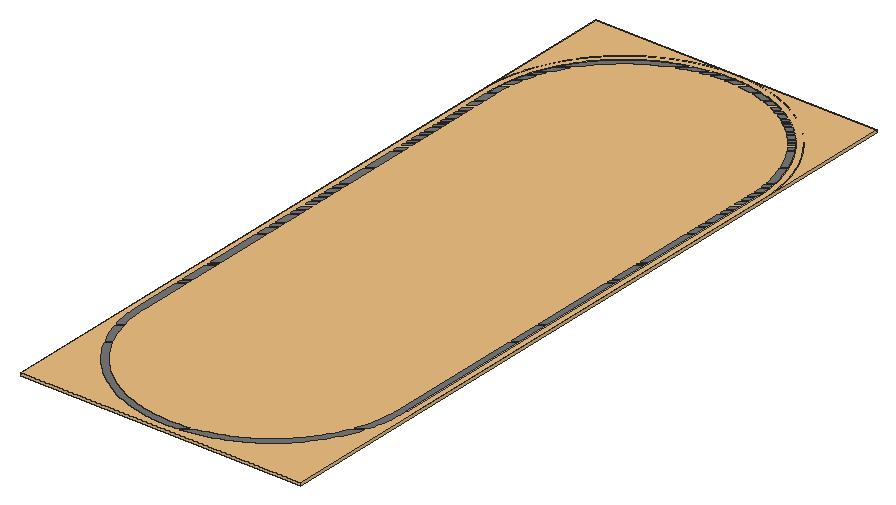
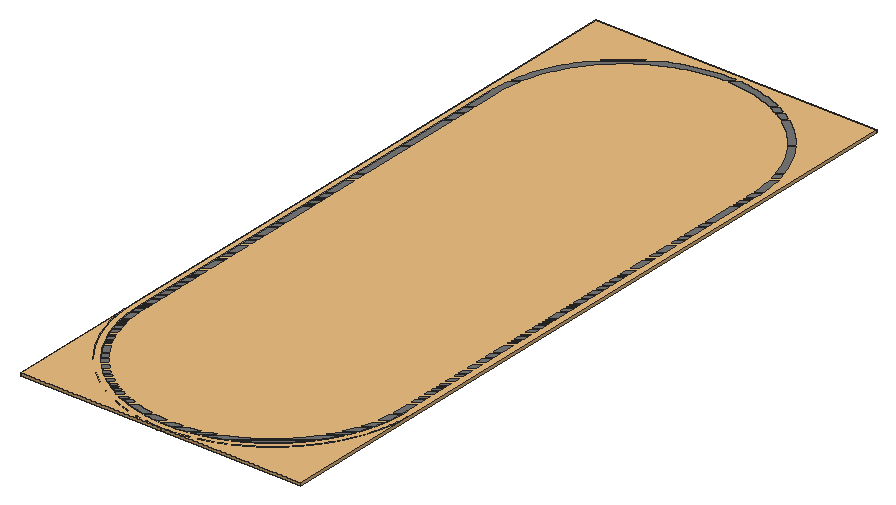
# SketchUp Ruby script. Lengths in inches.
U = 1.inch
M = Sketchup.active_model
def pt(a) = Geom::Point3d.new(a.map { |v| v * U })
def face(e, loops, mat)
  f = e.add_face(loops[0].map { |a| pt(a) })
  loops[1..].each { |l| e.add_face(l.map { |a| pt(a) }).erase! }
  f.material = f.back_material = mat if mat
  f
end
# faces: each face lists its corners as indices into pts; further lists are holes
def faces(e, pts, list, mat = nil) = list.each { |f| face(e, (f[0].is_a?(Array) ? f : [f]).map { |l| l.map { |i| pts[i] } }, mat) }
# xy, xz, yz: faces in a plane at the given z, y or x. An outline is a flat list of corners, or four numbers for a rectangle; further outlines are holes
def ring(l) = l.size == 4 ? [[l[0], l[1]], [l[2], l[1]], [l[2], l[3]], [l[0], l[3]]] : l.each_slice(2).to_a
def flat(e, list, mat, &to3) = list.each { |f| face(e, (f[0].is_a?(Array) ? f : [f]).map { |l| ring(l).map { |u, v| to3.(u, v) } }, mat) }
def xy(e, z, list, mat = nil) = flat(e, list, mat) { |x, y| [x, y, z] }
def xz(e, y, list, mat = nil) = flat(e, list, mat) { |x, z| [x, y, z] }
def yz(e, x, list, mat = nil) = flat(e, list, mat) { |y, z| [x, y, z] }
def lines(e, pts, list) = list.each { |a, b| e.add_line(pt(pts[a]), pt(pts[b])) }
# prism: a flat outline (further loops are holes) pulled along v
def prism(e, loops, v, mat = nil)
  f = face(e, loops, mat); d = Geom::Vector3d.new(v.map { |x| x * U })
  f.pushpull(f.normal.samedirection?(d) ? d.length : -d.length)
end
def box(e, o, s, mat = nil) = prism(e, [[o, [o[0] + s[0], o[1], o[2]], [o[0] + s[0], o[1] + s[1], o[2]], [o[0], o[1] + s[1], o[2]]]], [0, 0, s[2]], mat)
def at(x, y, z, deg = 0) = Geom::Transformation.translation(pt([x, y, z])) * Geom::Transformation.rotation(ORIGIN, Z_AXIS, deg.degrees)
def axes(o, x, y, z) = Geom::Transformation.new([*x, 0, *y, 0, *z, 0, *pt(o).to_a, 1])
def part(name) = M.definitions.add(name)
# library, detail: a bought-in or finely detailed component or shape, given as its bounding box
def library(name, o, s) = part(name).tap { |d| box(d.entities, o, s) }
def detail(e, o, s) = box(e.add_group.entities, o, s)
def put(e, d, t, mat = nil) = e.add_instance(d, t).tap { |i| i.material = mat if mat }
def group(e, t, mat = nil) = e.add_group.tap { |g| g.transformation = t; g.material = mat if mat }.entities
root = M.entities
M.materials.add("False ceiling Light").color = [253, 207, 127]
M.materials.add("[Slate Light Tile]").color = [119, 119, 119]
c1 = library("Group\#44",[0,0,0],[46,118,0.5])
xy(root,3,[[[189,26,189.58,26.01,190.15,26.03,190.73,26.07,191.3,26.12,191.87,26.1875,192.44,26.27,193.01,26.37,193.57,26.48,194.14,26.61,194.69,26.75,195.25,26.91,195.8,27.08,196.34,27.26,196.88,27.46,197.42,27.67,197.95,27.9,198.47,28.14,198.99,28.4,199.5,28.67,200,28.95,200.49,29.24,200.98,29.55,201.46,29.87,201.93,30.2,202.85,30.9,203.29,31.27,203.72,31.65,204.14,32.04,204.56,32.44,204.96,32.86,205.35,33.28,205.73,33.71,206.1,34.15,206.8,35.07,207.13,35.54,207.45,36.02,207.76,36.51,208.05,37,208.33,37.5,208.6,38.01,208.86,38.53,209.1,39.05,209.33,39.58,209.54,40.12,209.74,40.66,209.92,41.2,210.09,41.75,210.25,42.31,210.39,42.86,210.52,43.43,210.63,43.99,210.73,44.56,210.8125,45.13,210.88,45.7,210.93,46.27,210.97,46.85,210.99,47.42,211,48,211,120,210.99,120.58,210.97,121.15,210.93,121.73,210.88,122.3,210.8125,122.87,210.73,123.44,210.63,124.01,210.52,124.57,210.39,125.14,210.25,125.69,210.09,126.25,209.92,126.8,209.74,127.34,209.54,127.88,209.33,128.42,209.1,128.95,208.86,129.47,208.6,129.99,208.33,130.5,208.05,131,207.76,131.49,207.45,131.98,207.13,132.46,206.8,132.93,206.1,133.85,205.73,134.29,205.35,134.72,204.96,135.14,204.56,135.56,204.14,135.96,203.72,136.35,203.29,136.73,202.85,137.1,201.93,137.8,201.46,138.13,200.98,138.45,200.49,138.76,200,139.05,199.5,139.33,198.99,139.6,198.47,139.86,197.95,140.1,197.42,140.33,196.88,140.54,196.34,140.74,195.8,140.92,195.25,141.09,194.69,141.25,194.14,141.39,193.57,141.52,193.01,141.63,192.44,141.73,191.87,141.8125,191.3,141.88,190.73,141.93,190.15,141.97,189.58,141.99,189,142,188.42,141.99,187.85,141.97,187.27,141.93,186.7,141.88,186.13,141.8125,185.56,141.73,184.99,141.63,184.43,141.52,183.86,141.39,183.31,141.25,182.75,141.09,182.2,140.92,181.66,140.74,181.12,140.54,180.58,140.33,180.05,140.1,179.53,139.86,179.01,139.6,178.5,139.33,178,139.05,177.51,138.76,177.02,138.45,176.54,138.13,176.07,137.8,175.15,137.1,174.71,136.73,174.28,136.35,173.86,135.96,173.44,135.56,173.04,135.14,172.65,134.72,172.27,134.29,171.9,133.85,171.2,132.93,170.87,132.46,170.55,131.98,170.24,131.49,169.95,131,169.67,130.5,169.4,129.99,169.14,129.47,168.9,128.95,168.67,128.42,168.46,127.88,168.26,127.34,168.08,126.8,167.91,126.25,167.75,125.69,167.61,125.14,167.48,124.57,167.37,124.01,167.27,123.44,167.1875,122.87,167.12,122.3,167.07,121.73,167.03,121.15,167.01,120.58,167,120,167,48,167.01,47.42,167.03,46.85,167.07,46.27,167.12,45.7,167.1875,45.13,167.27,44.56,167.37,43.99,167.48,43.43,167.61,42.86,167.75,42.31,167.91,41.75,168.08,41.2,168.26,40.66,168.46,40.12,168.67,39.58,168.9,39.05,169.14,38.53,169.4,38.01,169.67,37.5,169.95,37,170.24,36.51,170.55,36.02,170.87,35.54,171.2,35.07,171.9,34.15,172.27,33.71,172.65,33.28,173.04,32.86,173.44,32.44,173.86,32.04,174.28,31.65,174.71,31.27,175.15,30.9,176.07,30.2,176.54,29.87,177.02,29.55,177.51,29.24,178,28.95,178.5,28.67,179.01,28.4,179.53,28.14,180.05,27.9,180.58,27.67,181.12,27.46,181.66,27.26,182.2,27.08,182.75,26.91,183.31,26.75,183.86,26.61,184.43,26.48,184.99,26.37,185.56,26.27,186.13,26.1875,186.7,26.12,187.27,26.07,187.85,26.03,188.42,26.01],[189,27,188.45,27.01,187.9,27.03,187.35,27.06,186.8,27.12,186.26,27.18,185.71,27.26,185.17,27.35,184.63,27.46,184.1,27.58,183.56,27.72,183.04,27.86,182.51,28.03,181.99,28.2,181.47,28.39,180.96,28.6,180.46,28.82,179.96,29.05,179.47,29.29,178.98,29.54,178.5,29.8125,178.03,30.09,177.5625,30.39,177.11,30.69,176.66,31.01,176.22,31.34,175.78,31.68,175.36,32.03,174.95,32.39,174.54,32.77,174.15,33.15,173.77,33.54,173.39,33.95,173.03,34.36,172.68,34.78,172.34,35.22,172.01,35.66,171.69,36.11,171.39,36.5625,171.09,37.03,170.8125,37.5,170.54,37.98,170.29,38.47,170.05,38.96,169.82,39.46,169.6,39.96,169.39,40.47,169.2,40.99,169.03,41.51,168.86,42.04,168.72,42.56,168.58,43.1,168.46,43.63,168.35,44.17,168.26,44.71,168.18,45.26,168.12,45.8,168.06,46.35,168.03,46.9,168.01,47.45,168,48,168,120,168.01,120.55,168.03,121.1,168.06,121.65,168.12,122.2,168.18,122.74,168.26,123.29,168.35,123.83,168.46,124.37,168.58,124.9,168.72,125.44,168.86,125.96,169.03,126.49,169.2,127.01,169.39,127.53,169.6,128.04,169.82,128.54,170.05,129.04,170.29,129.53,170.54,130.02,170.8125,130.5,171.09,130.97,171.39,131.4375,171.69,131.89,172.01,132.34,172.34,132.78,172.68,133.22,173.03,133.64,173.39,134.05,173.77,134.46,174.15,134.85,174.54,135.23,174.95,135.61,175.36,135.97,175.78,136.32,176.22,136.66,176.66,136.99,177.11,137.31,177.5625,137.61,178.03,137.91,178.5,138.1875,178.98,138.46,179.47,138.71,179.96,138.95,180.46,139.18,180.96,139.4,181.47,139.61,181.99,139.8,182.51,139.97,183.04,140.14,183.56,140.28,184.1,140.42,184.63,140.54,185.17,140.65,185.71,140.74,186.26,140.82,186.8,140.88,187.35,140.94,187.9,140.97,188.45,140.99,189,141,189.55,140.99,190.1,140.97,190.65,140.94,191.2,140.88,191.74,140.82,192.29,140.74,192.83,140.65,193.37,140.54,193.9,140.42,194.44,140.28,194.96,140.14,195.49,139.97,196.01,139.8,196.53,139.61,197.04,139.4,197.54,139.18,198.04,138.95,198.53,138.71,199.02,138.46,199.5,138.1875,199.97,137.91,200.4375,137.61,200.89,137.31,201.34,136.99,201.78,136.66,202.22,136.32,202.64,135.97,203.05,135.61,203.46,135.23,203.85,134.85,204.23,134.46,204.61,134.05,204.97,133.64,205.32,133.22,205.66,132.78,205.99,132.34,206.31,131.89,206.61,131.4375,206.91,130.97,207.1875,130.5,207.46,130.02,207.71,129.53,207.95,129.04,208.18,128.54,208.4,128.04,208.61,127.53,208.8,127.01,208.97,126.49,209.14,125.96,209.28,125.44,209.42,124.9,209.54,124.37,209.65,123.83,209.74,123.29,209.82,122.74,209.88,122.2,209.94,121.65,209.97,121.1,209.99,120.55,210,120,210,48,209.99,47.45,209.97,46.9,209.94,46.35,209.88,45.8,209.82,45.26,209.74,44.71,209.65,44.17,209.54,43.63,209.42,43.1,209.28,42.56,209.14,42.04,208.97,41.51,208.8,40.99,208.61,40.47,208.4,39.96,208.18,39.46,207.95,38.96,207.71,38.47,207.46,37.98,207.1875,37.5,206.91,37.03,206.61,36.5625,206.31,36.11,205.99,35.66,205.66,35.22,205.32,34.78,204.97,34.36,204.61,33.95,204.23,33.54,203.85,33.15,203.46,32.77,203.05,32.39,202.64,32.03,202.22,31.68,201.78,31.34,201.34,31.01,200.89,30.69,200.4375,30.39,199.97,30.09,199.5,29.8125,199.02,29.54,198.53,29.29,198.04,29.05,197.54,28.82,197.04,28.6,196.53,28.39,196.01,28.2,195.49,28.03,194.96,27.86,194.44,27.72,193.9,27.58,193.37,27.46,192.83,27.35,192.29,27.26,191.74,27.18,191.2,27.12,190.65,27.06,190.1,27.03,189.55,27.01]]],"[Slate Light Tile]")
yz(root,211,[[48,2.5,120,3]])
yz(root,212,[[48,2.5,120,3]])
p = [[166.01,120.6,3],[166,120,3],[166,120,2.5],[166.01,120.6,2.5],[167,120,3],[167.01,120.58,3],
  [167.01,120.58,2.5],[167,120,2.5],[210.99,120.58,3],[211,120,3],[211,120,2.5],[210.99,120.58,2.5],
  [212,120,3],[211.99,120.6,3],[211.99,120.6,2.5],[212,120,2.5],[166.03,121.2,3],[166.03,121.2,2.5],
  [167.03,121.15,3],[167.03,121.15,2.5],[210.97,121.15,3],[210.97,121.15,2.5],[211.97,121.2,3],[211.97,121.2,2.5],
  [166.07,121.8,3],[166.07,121.8,2.5],[167.07,121.73,3],[167.07,121.73,2.5],[210.93,121.73,3],[210.93,121.73,2.5],
  [211.93,121.8,3],[211.93,121.8,2.5],[167.12,122.3,3],[167.12,122.3,2.5],[210.88,122.3,3],[210.88,122.3,2.5],
  [166.125,122.4,3],[166.125,122.4,2.5],[211.875,122.4,3],[211.875,122.4,2.5],[167.1875,122.87,3],[167.1875,122.87,2.5],
  [210.8125,122.87,3],[210.8125,122.87,2.5],[166.2,123,3],[166.2,123,2.5],[211.8,123,3],[211.8,123,2.5],
  [167.27,123.44,3],[167.27,123.44,2.5],[210.73,123.44,3],[210.73,123.44,2.5],[166.28,123.6,3],[166.28,123.6,2.5],
  [211.72,123.6,3],[211.72,123.6,2.5],[167.37,124.01,3],[167.37,124.01,2.5],[210.63,124.01,3],[210.63,124.01,2.5],
  [166.39,124.19,3],[166.39,124.19,2.5],[211.61,124.19,3],[211.61,124.19,2.5],[167.48,124.57,3],[167.48,124.57,2.5],
  [210.52,124.57,3],[210.52,124.57,2.5],[166.5,124.78,3],[166.5,124.78,2.5],[211.5,124.78,3],[211.5,124.78,2.5],
  [167.61,125.14,3],[167.61,125.14,2.5],[210.39,125.14,3],[210.39,125.14,2.5],[166.64,125.37,3],[166.64,125.37,2.5],
  [211.36,125.37,3],[211.36,125.37,2.5],[167.75,125.69,3],[167.75,125.69,2.5],[210.25,125.69,3],[210.25,125.69,2.5],
  [166.78,125.95,3],[166.78,125.95,2.5],[211.22,125.95,3],[211.22,125.95,2.5],[167.91,126.25,3],[167.91,126.25,2.5],
  [210.09,126.25,3],[210.09,126.25,2.5],[166.95,126.53,3],[166.95,126.53,2.5],[211.05,126.53,3],[211.05,126.53,2.5],
  [168.08,126.8,3],[168.08,126.8,2.5],[209.92,126.8,3],[209.92,126.8,2.5],[167.125,127.11,3],[167.125,127.11,2.5],
  [210.875,127.11,3],[210.875,127.11,2.5],[168.26,127.34,3],[168.26,127.34,2.5],[209.74,127.34,3],[209.74,127.34,2.5],
  [167.32,127.68,3],[167.32,127.68,2.5],[210.68,127.68,3],[210.68,127.68,2.5],[168.46,127.88,3],[168.46,127.88,2.5],
  [209.54,127.88,3],[209.54,127.88,2.5],[167.53,128.24,3],[167.53,128.24,2.5],[210.47,128.24,3],[210.47,128.24,2.5],
  [168.67,128.42,3],[168.67,128.42,2.5],[209.33,128.42,3],[209.33,128.42,2.5],[167.75,128.8,3],[167.75,128.8,2.5],
  [210.25,128.8,3],[210.25,128.8,2.5],[168.9,128.95,3],[168.9,128.95,2.5],[209.1,128.95,3],[209.1,128.95,2.5],
  [167.99,129.35,3],[167.99,129.35,2.5],[210.01,129.35,3],[210.01,129.35,2.5],[169.14,129.47,3],[169.14,129.47,2.5],
  [208.86,129.47,3],[208.86,129.47,2.5],[168.24,129.9,3],[168.24,129.9,2.5],[209.76,129.9,3],[209.76,129.9,2.5],
  [169.4,129.99,3],[169.4,129.99,2.5],[208.6,129.99,3],[208.6,129.99,2.5],[168.51,130.44,3],[168.51,130.44,2.5],
  [209.49,130.44,3],[209.49,130.44,2.5],[169.67,130.5,3],[169.67,130.5,2.5],[208.33,130.5,3],[208.33,130.5,2.5],
  [168.79,130.97,3],[168.79,130.97,2.5],[209.21,130.97,3],[209.21,130.97,2.5],[169.95,131,3],[169.95,131,2.5],
  [208.05,131,3],[208.05,131,2.5],[169.08,131.5,3],[169.08,131.5,2.5],[170.24,131.49,3],[170.24,131.49,2.5],
  [207.76,131.49,3],[207.76,131.49,2.5],[208.92,131.5,3],[208.92,131.5,2.5],[169.39,132.02,3],[169.39,132.02,2.5],
  [170.55,131.98,3],[170.55,131.98,2.5],[207.45,131.98,3],[207.45,131.98,2.5],[208.61,132.02,3],[208.61,132.02,2.5],
  [169.71,132.53,3],[169.71,132.53,2.5],[170.87,132.46,3],[170.87,132.46,2.5],[207.13,132.46,3],[207.13,132.46,2.5],
  [208.29,132.53,3],[208.29,132.53,2.5],[170.05,133.03,3],[170.05,133.03,2.5],[171.2,132.93,3],[171.2,132.93,2.5],
  [206.8,132.93,3],[206.8,132.93,2.5],[207.95,133.03,3],[207.95,133.03,2.5],[171.55,133.39,3],[171.55,133.39,2.5],
  [206.45,133.39,3],[206.45,133.39,2.5],[170.39,133.52,3],[170.39,133.52,2.5],[207.61,133.52,3],[207.61,133.52,2.5],
  [171.9,133.85,3],[171.9,133.85,2.5],[206.1,133.85,3],[206.1,133.85,2.5],[170.75,134,3],[170.75,134,2.5],
  [207.25,134,3],[207.25,134,2.5],[172.27,134.29,3],[172.27,134.29,2.5],[205.73,134.29,3],[205.73,134.29,2.5],
  [171.125,134.47,3],[171.125,134.47,2.5],[206.875,134.47,3],[206.875,134.47,2.5],[172.65,134.72,3],[172.65,134.72,2.5],
  [205.35,134.72,3],[205.35,134.72,2.5],[171.51,134.9375,3],[171.51,134.9375,2.5],[206.49,134.9375,3],[206.49,134.9375,2.5],
  [173.04,135.14,3],[173.04,135.14,2.5],[204.96,135.14,3],[204.96,135.14,2.5],[171.91,135.39,3],[171.91,135.39,2.5],
  [206.09,135.39,3],[206.09,135.39,2.5],[173.44,135.56,3],[173.44,135.56,2.5],[204.56,135.56,3],[204.56,135.56,2.5],
  [172.32,135.83,3],[172.32,135.83,2.5],[205.68,135.83,3],[205.68,135.83,2.5],[173.86,135.96,3],[173.86,135.96,2.5],
  [204.14,135.96,3],[204.14,135.96,2.5],[172.74,136.26,3],[172.74,136.26,2.5],[205.26,136.26,3],[205.26,136.26,2.5],
  [174.28,136.35,3],[174.28,136.35,2.5],[203.72,136.35,3],[203.72,136.35,2.5],[173.17,136.68,3],[173.17,136.68,2.5],
  [174.71,136.73,3],[174.71,136.73,2.5],[203.29,136.73,3],[203.29,136.73,2.5],[204.83,136.68,3],[204.83,136.68,2.5],
  [173.61,137.09,3],[173.61,137.09,2.5],[175.15,137.1,3],[175.15,137.1,2.5],[202.85,137.1,3],[202.85,137.1,2.5],
  [204.39,137.09,3],[204.39,137.09,2.5],[174.0625,137.49,3],[174.0625,137.49,2.5],[175.61,137.45,3],[175.61,137.45,2.5],
  [202.39,137.45,3],[202.39,137.45,2.5],[203.9375,137.49,3],[203.9375,137.49,2.5],[174.53,137.875,3],[174.53,137.875,2.5],
  [176.07,137.8,3],[176.07,137.8,2.5],[201.93,137.8,3],[201.93,137.8,2.5],[203.47,137.875,3],[203.47,137.875,2.5],
  [176.54,138.13,3],[176.54,138.13,2.5],[201.46,138.13,3],[201.46,138.13,2.5],[175,138.25,3],[175,138.25,2.5],
  [203,138.25,3],[203,138.25,2.5],[177.02,138.45,3],[177.02,138.45,2.5],[200.98,138.45,3],[200.98,138.45,2.5],
  [175.48,138.61,3],[175.48,138.61,2.5],[202.52,138.61,3],[202.52,138.61,2.5],[177.51,138.76,3],[177.51,138.76,2.5],
  [200.49,138.76,3],[200.49,138.76,2.5],[175.97,138.95,3],[175.97,138.95,2.5],[202.03,138.95,3],[202.03,138.95,2.5],
  [178,139.05,3],[178,139.05,2.5],[200,139.05,3],[200,139.05,2.5],[176.47,139.29,3],[176.47,139.29,2.5],
  [201.53,139.29,3],[201.53,139.29,2.5],[178.5,139.33,3],[178.5,139.33,2.5],[199.5,139.33,3],[199.5,139.33,2.5],
  [176.98,139.61,3],[176.98,139.61,2.5],[179.01,139.6,3],[179.01,139.6,2.5],[198.99,139.6,3],[198.99,139.6,2.5],
  [201.02,139.61,3],[201.02,139.61,2.5],[177.5,139.92,3],[177.5,139.92,2.5],[179.53,139.86,3],[179.53,139.86,2.5],
  [198.47,139.86,3],[198.47,139.86,2.5],[200.5,139.92,3],[200.5,139.92,2.5],[178.03,140.21,3],[178.03,140.21,2.5],
  [180.05,140.1,3],[180.05,140.1,2.5],[197.95,140.1,3],[197.95,140.1,2.5],[199.97,140.21,3],[199.97,140.21,2.5],
  [180.58,140.33,3],[180.58,140.33,2.5],[197.42,140.33,3],[197.42,140.33,2.5],[178.56,140.49,3],[178.56,140.49,2.5],
  [199.44,140.49,3],[199.44,140.49,2.5],[181.12,140.54,3],[181.12,140.54,2.5],[196.88,140.54,3],[196.88,140.54,2.5],
  [179.1,140.76,3],[179.1,140.76,2.5],[181.66,140.74,3],[181.66,140.74,2.5],[196.34,140.74,3],[196.34,140.74,2.5],
  [198.9,140.76,3],[198.9,140.76,2.5],[182.2,140.92,3],[182.2,140.92,2.5],[195.8,140.92,3],[195.8,140.92,2.5],
  [179.65,141.01,3],[179.65,141.01,2.5],[198.35,141.01,3],[198.35,141.01,2.5],[182.75,141.09,3],[182.75,141.09,2.5],
  [195.25,141.09,3],[195.25,141.09,2.5],[180.2,141.25,3],[180.2,141.25,2.5],[197.8,141.25,3],[197.8,141.25,2.5],
  [183.31,141.25,3],[183.31,141.25,2.5],[194.69,141.25,3],[194.69,141.25,2.5],[180.76,141.47,3],[180.76,141.47,2.5],
  [197.24,141.47,3],[197.24,141.47,2.5],[183.86,141.39,3],[183.86,141.39,2.5],[194.14,141.39,3],[194.14,141.39,2.5],
  [184.43,141.52,3],[184.43,141.52,2.5],[193.57,141.52,3],[193.57,141.52,2.5],[181.32,141.68,3],[181.32,141.68,2.5],
  [184.99,141.63,3],[184.99,141.63,2.5],[193.01,141.63,3],[193.01,141.63,2.5],[196.68,141.68,3],[196.68,141.68,2.5],
  [185.56,141.73,3],[185.56,141.73,2.5],[192.44,141.73,3],[192.44,141.73,2.5],[181.89,141.875,3],[181.89,141.875,2.5],
  [186.13,141.8125,3],[186.13,141.8125,2.5],[191.87,141.8125,3],[191.87,141.8125,2.5],[196.11,141.875,3],[196.11,141.875,2.5],
  [186.7,141.88,3],[186.7,141.88,2.5],[191.3,141.88,3],[191.3,141.88,2.5],[182.47,142.05,3],[182.47,142.05,2.5],
  [187.27,141.93,3],[187.27,141.93,2.5],[187.85,141.97,3],[187.85,141.97,2.5],[190.15,141.97,3],[190.73,141.93,3],
  [190.73,141.93,2.5],[190.15,141.97,2.5],[195.53,142.05,3],[195.53,142.05,2.5],[188.42,141.99,3],[188.42,141.99,2.5],
  [189,142,3],[189,142,2.5],[189.58,141.99,3],[189.58,141.99,2.5],[183.05,142.22,3],[183.05,142.22,2.5],
  [194.95,142.22,3],[194.95,142.22,2.5],[183.63,142.36,3],[183.63,142.36,2.5],[194.37,142.36,3],[194.37,142.36,2.5],
  [184.22,142.5,3],[184.22,142.5,2.5],[193.78,142.5,3],[193.78,142.5,2.5],[184.81,142.61,3],[184.81,142.61,2.5],
  [193.19,142.61,3],[193.19,142.61,2.5],[185.4,142.72,3],[185.4,142.72,2.5],[192.6,142.72,3],[192.6,142.72,2.5],
  [186,142.8,3],[186,142.8,2.5],[192,142.8,3],[192,142.8,2.5],[186.6,142.875,3],[186.6,142.875,2.5],
  [191.4,142.875,3],[191.4,142.875,2.5],[187.2,142.93,3],[187.2,142.93,2.5],[187.8,142.97,3],[187.8,142.97,2.5],
  [190.8,142.93,3],[190.2,142.97,3],[190.2,142.97,2.5],[190.8,142.93,2.5],[188.4,142.99,3],[188.4,142.99,2.5],
  [189,143,3],[189,143,2.5],[189.6,142.99,3],[189.6,142.99,2.5]]
faces(root,p,[[0,1,2,3],[4,5,6,7],[8,9,10,11],[12,13,14,15],[16,0,3,17],[5,18,19,6],[20,8,11,21],[13,22,23,14],
  [24,16,17,25],[18,26,27,19],[28,20,21,29],[22,30,31,23],[26,32,33,27],[34,28,29,35],[36,24,25,37],[30,38,39,31],
  [32,40,41,33],[42,34,35,43],[44,36,37,45],[38,46,47,39],[40,48,49,41],[50,42,43,51],[52,44,45,53],[46,54,55,47],
  [48,56,57,49],[58,50,51,59],[60,52,53,61],[54,62,63,55],[56,64,65,57],[66,58,59,67],[68,60,61,69],[62,70,71,63],
  [64,72,73,65],[74,66,67,75],[76,68,69,77],[70,78,79,71],[72,80,81,73],[82,74,75,83],[84,76,77,85],[78,86,87,79],
  [80,88,89,81],[90,82,83,91],[92,84,85,93],[86,94,95,87],[88,96,97,89],[98,90,91,99],[100,92,93,101],[94,102,103,95],
  [96,104,105,97],[106,98,99,107],[108,100,101,109],[102,110,111,103],[104,112,113,105],[114,106,107,115],[116,108,109,117],[110,118,119,111],
  [112,120,121,113],[122,114,115,123],[124,116,117,125],[118,126,127,119],[120,128,129,121],[130,122,123,131],[132,124,125,133],[126,134,135,127],
  [128,136,137,129],[138,130,131,139],[140,132,133,141],[134,142,143,135],[136,144,145,137],[146,138,139,147],[148,140,141,149],[142,150,151,143],
  [144,152,153,145],[154,146,147,155],[156,148,149,157],[150,158,159,151],[152,160,161,153],[162,154,155,163],[164,156,157,165],[160,166,167,161],
  [168,162,163,169],[158,170,171,159],[172,164,165,173],[166,174,175,167],[176,168,169,177],[170,178,179,171],[180,172,173,181],[174,182,183,175],
  [184,176,177,185],[178,186,187,179],[188,180,181,189],[182,190,191,183],[192,184,185,193],[186,194,195,187],[190,196,197,191],[198,192,193,199],
  [200,188,189,201],[194,202,203,195],[196,204,205,197],[206,198,199,207],[208,200,201,209],[202,210,211,203],[204,212,213,205],[214,206,207,215],
  [216,208,209,217],[210,218,219,211],[212,220,221,213],[222,214,215,223],[224,216,217,225],[218,226,227,219],[220,228,229,221],[230,222,223,231],
  [232,224,225,233],[226,234,235,227],[228,236,237,229],[238,230,231,239],[240,232,233,241],[234,242,243,235],[236,244,245,237],[246,238,239,247],
  [248,240,241,249],[242,250,251,243],[244,252,253,245],[254,246,247,255],[256,248,249,257],[252,258,259,253],[260,254,255,261],[250,262,263,251],
  [264,256,257,265],[258,266,267,259],[268,260,261,269],[262,270,271,263],[272,264,265,273],[266,274,275,267],[276,268,269,277],[270,278,279,271],
  [280,272,273,281],[274,282,283,275],[284,276,277,285],[278,286,287,279],[282,288,289,283],[290,284,285,291],[292,280,281,293],[286,294,295,287],
  [288,296,297,289],[298,290,291,299],[300,292,293,301],[294,302,303,295],[296,304,305,297],[306,298,299,307],[308,300,301,309],[302,310,311,303],
  [304,312,313,305],[314,306,307,315],[316,308,309,317],[310,318,319,311],[312,320,321,313],[322,314,315,323],[324,316,317,325],[320,326,327,321],
  [328,322,323,329],[318,330,331,319],[332,324,325,333],[326,334,335,327],[336,328,329,337],[330,338,339,331],[340,332,333,341],[334,342,343,335],
  [344,336,337,345],[338,346,347,339],[342,348,349,343],[350,344,345,351],[352,340,341,353],[346,354,355,347],[348,356,357,349],[358,350,351,359],
  [360,352,353,361],[356,362,363,357],[364,358,359,365],[354,366,367,355],[362,368,369,363],[370,364,365,371],[372,360,361,373],[366,374,375,367],
  [368,376,377,369],[378,370,371,379],[380,372,373,381],[374,382,383,375],[376,384,385,377],[386,378,379,387],[388,380,381,389],[382,390,391,383],
  [384,392,393,385],[394,386,387,395],[392,396,397,393],[398,394,395,399],[400,388,389,401],[396,402,403,397],[404,398,399,405],[390,406,407,391],
  [402,408,409,403],[410,404,405,411],[412,400,401,413],[408,414,415,409],[416,410,411,417],[406,418,419,407],[414,420,421,415],[422,416,417,423],
  [424,412,413,425],[420,426,427,421],[426,428,429,427],[430,431,432,433],[431,422,423,432],[418,434,435,419],[428,436,437,429],[436,438,439,437],
  [438,440,441,439],[440,430,433,441],[442,424,425,443],[434,444,445,435],[446,442,443,447],[444,448,449,445],[450,446,447,451],[448,452,453,449],
  [454,450,451,455],[452,456,457,453],[458,454,455,459],[456,460,461,457],[462,458,459,463],[460,464,465,461],[466,462,463,467],[464,468,469,465],
  [470,466,467,471],[472,470,471,473],[474,475,476,477],[468,474,477,469],[478,472,473,479],[480,478,479,481],[482,480,481,483],[475,482,483,476]])
put(root,c1,at(166,25,2.5),"False ceiling Light")
